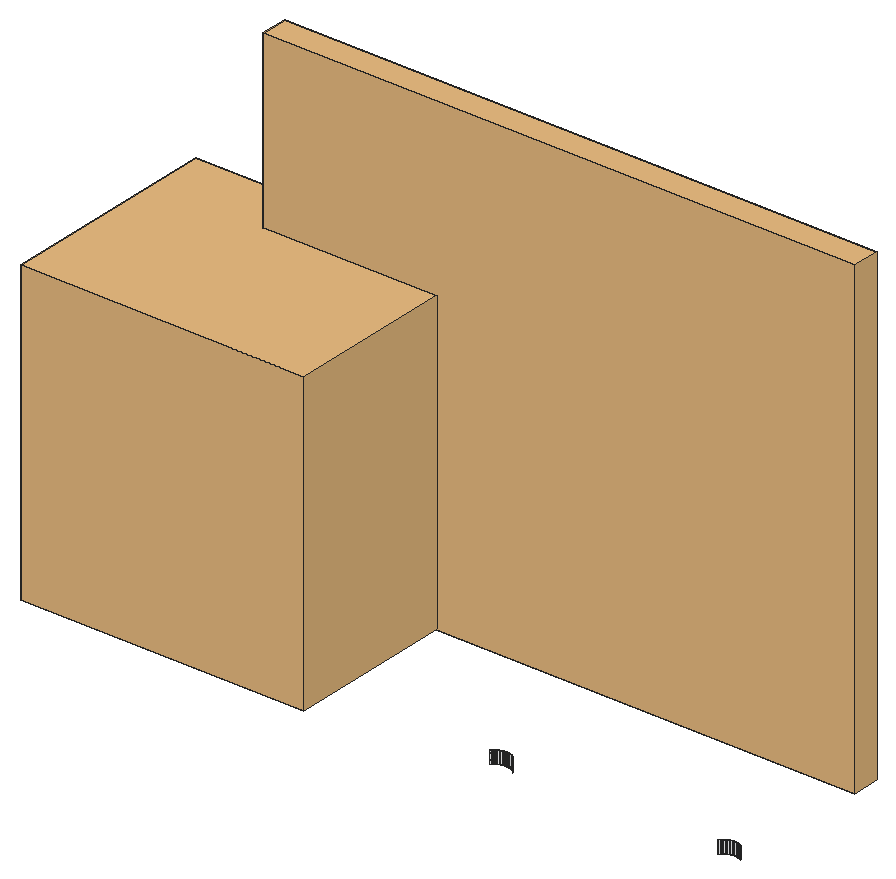
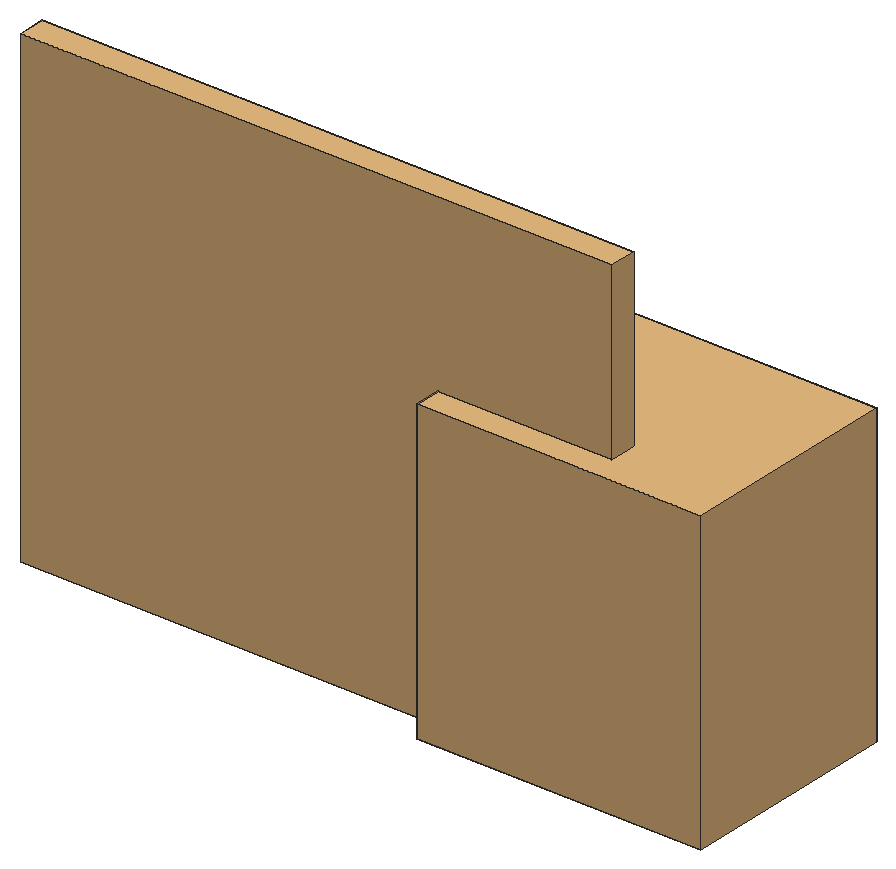
# SketchUp Ruby script. Lengths in inches.
U = 1.inch
M = Sketchup.active_model
def pt(a) = Geom::Point3d.new(a.map { |v| v * U })
def face(e, loops, mat)
  f = e.add_face(loops[0].map { |a| pt(a) })
  loops[1..].each { |l| e.add_face(l.map { |a| pt(a) }).erase! }
  f.material = f.back_material = mat if mat
  f
end
# faces: each face lists its corners as indices into pts; further lists are holes
def faces(e, pts, list, mat = nil) = list.each { |f| face(e, (f[0].is_a?(Array) ? f : [f]).map { |l| l.map { |i| pts[i] } }, mat) }
# xy, xz, yz: faces in a plane at the given z, y or x. An outline is a flat list of corners, or four numbers for a rectangle; further outlines are holes
def ring(l) = l.size == 4 ? [[l[0], l[1]], [l[2], l[1]], [l[2], l[3]], [l[0], l[3]]] : l.each_slice(2).to_a
def flat(e, list, mat, &to3) = list.each { |f| face(e, (f[0].is_a?(Array) ? f : [f]).map { |l| ring(l).map { |u, v| to3.(u, v) } }, mat) }
def xy(e, z, list, mat = nil) = flat(e, list, mat) { |x, y| [x, y, z] }
def xz(e, y, list, mat = nil) = flat(e, list, mat) { |x, z| [x, y, z] }
def yz(e, x, list, mat = nil) = flat(e, list, mat) { |y, z| [x, y, z] }
def lines(e, pts, list) = list.each { |a, b| e.add_line(pt(pts[a]), pt(pts[b])) }
# prism: a flat outline (further loops are holes) pulled along v
def prism(e, loops, v, mat = nil)
  f = face(e, loops, mat); d = Geom::Vector3d.new(v.map { |x| x * U })
  f.pushpull(f.normal.samedirection?(d) ? d.length : -d.length)
end
def box(e, o, s, mat = nil) = prism(e, [[o, [o[0] + s[0], o[1], o[2]], [o[0] + s[0], o[1] + s[1], o[2]], [o[0], o[1] + s[1], o[2]]]], [0, 0, s[2]], mat)
def at(x, y, z, deg = 0) = Geom::Transformation.translation(pt([x, y, z])) * Geom::Transformation.rotation(ORIGIN, Z_AXIS, deg.degrees)
def axes(o, x, y, z) = Geom::Transformation.new([*x, 0, *y, 0, *z, 0, *pt(o).to_a, 1])
def part(name) = M.definitions.add(name)
# library, detail: a bought-in or finely detailed component or shape, given as its bounding box
def library(name, o, s) = part(name).tap { |d| box(d.entities, o, s) }
def detail(e, o, s) = box(e.add_group.entities, o, s)
def put(e, d, t, mat = nil) = e.add_instance(d, t).tap { |i| i.material = mat if mat }
def group(e, t, mat = nil) = e.add_group.tap { |g| g.transformation = t; g.material = mat if mat }.entities
root = M.entities
M.materials.add("[Metal Seamed]").color = [36, 36, 35]
M.materials.add("[Quartz Light Grey]").color = [251, 251, 252]
c1 = library("aaa",[130.5625,121.2,0],[57.57,44.48,60.75])
c2 = library("Group\#8",[0,-4.15,0],[120,5.53,96])
xz(root,256,[[68.84,117,68.92,119.5],[68.92,117,69,119.5],[69,117,69.08,119.5],[69.08,117,69.16,119.5],[115.18,117,115.25,119.5],
  [115.25,117,115.33,119.5],[115.33,117,115.41,119.5],[115.41,117,115.49,119.5],[161.51,117,161.59,119.5],[161.59,117,161.67,119.5],
  [161.67,117,161.75,119.5],[161.75,117,161.82,119.5]],"[Quartz Light Grey]")
p = [[66.62,254.83,117],[66.67,254.89,117],[66.67,254.89,119.5],[66.62,254.83,119.5],[71.33,254.89,117],[71.38,254.83,117],
  [71.38,254.83,119.5],[71.33,254.89,119.5],[112.95,254.83,117],[113,254.89,117],[113,254.89,119.5],[112.95,254.83,119.5],
  [117.66,254.89,117],[117.71,254.83,117],[117.71,254.83,119.5],[117.66,254.89,119.5],[159.29,254.83,117],[159.34,254.89,117],
  [159.34,254.89,119.5],[159.29,254.83,119.5],[66.72,254.95,117],[66.72,254.95,119.5],[66.77,255.01,117],[66.77,255.01,119.5],
  [71.23,255.01,117],[71.28,254.95,117],[71.28,254.95,119.5],[71.23,255.01,119.5],[113.05,254.95,117],[113.05,254.95,119.5],
  [113.1,255.01,117],[113.1,255.01,119.5],[117.5625,255.01,117],[117.61,254.95,117],[117.61,254.95,119.5],[117.5625,255.01,119.5],
  [159.39,254.95,117],[159.39,254.95,119.5],[159.4375,255.01,117],[159.4375,255.01,119.5],[66.82,255.07,117],[66.82,255.07,119.5],
  [71.18,255.07,117],[71.18,255.07,119.5],[113.16,255.07,117],[113.16,255.07,119.5],[117.51,255.07,117],[117.51,255.07,119.5],
  [159.49,255.07,117],[159.49,255.07,119.5],[66.88,255.12,117],[66.88,255.12,119.5],[66.93,255.18,117],[66.93,255.18,119.5],
  [71.07,255.18,117],[71.12,255.12,117],[71.12,255.12,119.5],[71.07,255.18,119.5],[113.21,255.12,117],[113.21,255.12,119.5],
  [113.27,255.18,117],[113.27,255.18,119.5],[117.4,255.18,117],[117.45,255.12,117],[117.45,255.12,119.5],[117.4,255.18,119.5],
  [159.55,255.12,117],[159.55,255.12,119.5],[159.6,255.18,117],[159.6,255.18,119.5],[66.99,255.23,117],[66.99,255.23,119.5],
  [67.05,255.28,117],[67.05,255.28,119.5],[70.95,255.28,117],[71.01,255.23,117],[71.01,255.23,119.5],[70.95,255.28,119.5],
  [113.33,255.23,117],[113.33,255.23,119.5],[113.38,255.28,117],[113.38,255.28,119.5],[117.28,255.28,117],[117.34,255.23,117],
  [117.34,255.23,119.5],[117.28,255.28,119.5],[159.66,255.23,117],[159.66,255.23,119.5],[159.72,255.28,117],[159.72,255.28,119.5],
  [67.11,255.33,117],[67.11,255.33,119.5],[67.17,255.38,117],[67.17,255.38,119.5],[70.83,255.38,117],[70.89,255.33,117],
  [70.89,255.33,119.5],[70.83,255.38,119.5],[113.45,255.33,117],[113.45,255.33,119.5],[113.51,255.38,117],[113.51,255.38,119.5],
  [117.16,255.38,117],[117.22,255.33,117],[117.22,255.33,119.5],[117.16,255.38,119.5],[159.78,255.33,117],[159.78,255.33,119.5],
  [159.84,255.38,117],[159.84,255.38,119.5],[67.24,255.43,117],[67.24,255.43,119.5],[67.3,255.47,117],[67.3,255.47,119.5],
  [70.7,255.47,117],[70.76,255.43,117],[70.76,255.43,119.5],[70.7,255.47,119.5],[113.57,255.43,117],[113.57,255.43,119.5],
  [113.63,255.47,117],[113.63,255.47,119.5],[117.03,255.47,117],[117.1,255.43,117],[117.1,255.43,119.5],[117.03,255.47,119.5],
  [159.9,255.43,117],[159.9,255.43,119.5],[159.97,255.47,117],[159.97,255.47,119.5],[67.37,255.52,117],[67.37,255.52,119.5],
  [67.43,255.56,117],[67.43,255.56,119.5],[70.57,255.56,117],[70.63,255.52,117],[70.63,255.52,119.5],[70.57,255.56,119.5],
  [113.7,255.52,117],[113.7,255.52,119.5],[113.77,255.56,117],[113.77,255.56,119.5],[116.9,255.56,117],[116.97,255.52,117],
  [116.97,255.52,119.5],[116.9,255.56,119.5],[160.03,255.52,117],[160.03,255.52,119.5],[160.1,255.56,117],[160.1,255.56,119.5],
  [163.23,255.56,117],[163.3,255.52,117],[163.3,255.52,119.5],[163.23,255.56,119.5],[67.5,255.6,117],[67.5,255.6,119.5],
  [67.57,255.64,117],[67.57,255.64,119.5],[67.64,255.67,117],[67.64,255.67,119.5],[70.36,255.67,117],[70.43,255.64,117],
  [70.43,255.64,119.5],[70.36,255.67,119.5],[70.5,255.6,117],[70.5,255.6,119.5],[113.83,255.6,117],[113.83,255.6,119.5],
  [113.9,255.64,117],[113.9,255.64,119.5],[113.97,255.67,117],[113.97,255.67,119.5],[116.7,255.67,117],[116.76,255.64,117],
  [116.76,255.64,119.5],[116.7,255.67,119.5],[116.83,255.6,117],[116.83,255.6,119.5],[160.17,255.6,117],[160.17,255.6,119.5],
  [160.24,255.64,117],[160.24,255.64,119.5],[160.3,255.67,117],[160.3,255.67,119.5],[163.03,255.67,117],[163.1,255.64,117],
  [163.1,255.64,119.5],[163.03,255.67,119.5],[163.17,255.6,117],[163.17,255.6,119.5],[67.71,255.71,117],[67.71,255.71,119.5],
  [67.78,255.74,117],[67.78,255.74,119.5],[67.85,255.77,117],[67.85,255.77,119.5],[70.15,255.77,117],[70.22,255.74,117],
  [70.22,255.74,119.5],[70.15,255.77,119.5],[70.29,255.71,117],[70.29,255.71,119.5],[114.04,255.71,117],[114.04,255.71,119.5],
  [114.11,255.74,117],[114.11,255.74,119.5],[114.19,255.77,117],[114.19,255.77,119.5],[116.48,255.77,117],[116.55,255.74,117],
  [116.55,255.74,119.5],[116.48,255.77,119.5],[116.625,255.71,117],[116.625,255.71,119.5],[160.375,255.71,117],[160.375,255.71,119.5],
  [160.45,255.74,117],[160.45,255.74,119.5],[160.52,255.77,117],[160.52,255.77,119.5],[162.81,255.77,117],[162.89,255.74,117],
  [162.89,255.74,119.5],[162.81,255.77,119.5],[162.96,255.71,117],[162.96,255.71,119.5],[67.92,255.8,117],[67.92,255.8,119.5],
  [68,255.83,117],[68,255.83,119.5],[68.07,255.85,117],[68.07,255.85,119.5],[69.93,255.85,117],[70,255.83,117],
  [70,255.83,119.5],[69.93,255.85,119.5],[70.08,255.8,117],[70.08,255.8,119.5],[114.26,255.8,117],[114.26,255.8,119.5],
  [114.33,255.83,117],[114.33,255.83,119.5],[114.41,255.85,117],[114.41,255.85,119.5],[116.26,255.85,117],[116.33,255.83,117],
  [116.33,255.83,119.5],[116.26,255.85,119.5],[116.41,255.8,117],[116.41,255.8,119.5],[160.59,255.8,117],[160.59,255.8,119.5],
  [160.67,255.83,117],[160.67,255.83,119.5],[160.74,255.85,117],[160.74,255.85,119.5],[162.59,255.85,117],[162.67,255.83,117],
  [162.67,255.83,119.5],[162.59,255.85,119.5],[162.74,255.8,117],[162.74,255.8,119.5],[68.15,255.875,117],[68.15,255.875,119.5],
  [68.22,255.9,117],[68.22,255.9,119.5],[68.3,255.92,117],[68.3,255.92,119.5],[68.375,255.93,117],[68.375,255.93,119.5],
  [68.45,255.95,117],[68.45,255.95,119.5],[68.53,255.96,117],[68.53,255.96,119.5],[69.47,255.96,117],[69.55,255.95,117],
  [69.55,255.95,119.5],[69.47,255.96,119.5],[69.625,255.93,117],[69.625,255.93,119.5],[69.7,255.92,117],[69.7,255.92,119.5],
  [69.78,255.9,117],[69.78,255.9,119.5],[69.85,255.875,117],[69.85,255.875,119.5],[114.48,255.875,117],[114.48,255.875,119.5],
  [114.56,255.9,117],[114.56,255.9,119.5],[114.63,255.92,117],[114.63,255.92,119.5],[114.71,255.93,117],[114.71,255.93,119.5],
  [114.79,255.95,117],[114.79,255.95,119.5],[114.86,255.96,117],[114.86,255.96,119.5],[115.8,255.96,117],[115.88,255.95,117],
  [115.88,255.95,119.5],[115.8,255.96,119.5],[115.96,255.93,117],[115.96,255.93,119.5],[116.03,255.92,117],[116.03,255.92,119.5],
  [116.11,255.9,117],[116.11,255.9,119.5],[116.19,255.875,117],[116.19,255.875,119.5],[160.81,255.875,117],[160.81,255.875,119.5],
  [160.89,255.9,117],[160.89,255.9,119.5],[160.97,255.92,117],[160.97,255.92,119.5],[161.04,255.93,117],[161.04,255.93,119.5],
  [161.12,255.95,117],[161.12,255.95,119.5],[161.2,255.96,117],[161.2,255.96,119.5],[162.14,255.96,117],[162.21,255.95,117],
  [162.21,255.95,119.5],[162.14,255.96,119.5],[162.29,255.93,117],[162.29,255.93,119.5],[162.37,255.92,117],[162.37,255.92,119.5],
  [162.44,255.9,117],[162.44,255.9,119.5],[162.52,255.875,117],[162.52,255.875,119.5],[68.61,255.97,117],[68.61,255.97,119.5],
  [68.6875,255.98,117],[68.6875,255.98,119.5],[68.76,255.99,117],[68.76,255.99,119.5],[68.84,256,117],[68.84,256,119.5],
  [69.16,256,117],[69.24,255.99,117],[69.24,255.99,119.5],[69.16,256,119.5],[69.3125,255.98,117],[69.3125,255.98,119.5],
  [69.39,255.97,117],[69.39,255.97,119.5],[114.94,255.97,117],[114.94,255.97,119.5],[115.02,255.98,117],[115.02,255.98,119.5],
  [115.1,255.99,117],[115.1,255.99,119.5],[115.18,256,117],[115.18,256,119.5],[115.49,256,117],[115.57,255.99,117],
  [115.57,255.99,119.5],[115.49,256,119.5],[115.65,255.98,117],[115.65,255.98,119.5],[115.72,255.97,117],[115.72,255.97,119.5],
  [161.28,255.97,117],[161.28,255.97,119.5],[161.35,255.98,117],[161.35,255.98,119.5],[161.43,255.99,117],[161.43,255.99,119.5],
  [161.51,256,117],[161.51,256,119.5],[161.82,256,117],[161.9,255.99,117],[161.9,255.99,119.5],[161.82,256,119.5],
  [161.98,255.98,117],[161.98,255.98,119.5],[162.06,255.97,117],[162.06,255.97,119.5],[54,271,126],[174,271,126]]
faces(root,p,[[0,1,2,3],[4,5,6,7],[8,9,10,11],[12,13,14,15],[16,17,18,19],[1,20,21,2],[20,22,23,21],[24,25,26,27],
  [25,4,7,26],[9,28,29,10],[28,30,31,29],[32,33,34,35],[33,12,15,34],[17,36,37,18],[36,38,39,37],[22,40,41,23],
  [42,24,27,43],[30,44,45,31],[46,32,35,47],[38,48,49,39],[40,50,51,41],[50,52,53,51],[54,55,56,57],[55,42,43,56],
  [44,58,59,45],[58,60,61,59],[62,63,64,65],[63,46,47,64],[48,66,67,49],[66,68,69,67],[52,70,71,53],[70,72,73,71],
  [74,75,76,77],[75,54,57,76],[60,78,79,61],[78,80,81,79],[82,83,84,85],[83,62,65,84],[68,86,87,69],[86,88,89,87],
  [72,90,91,73],[90,92,93,91],[94,95,96,97],[95,74,77,96],[80,98,99,81],[98,100,101,99],[102,103,104,105],[103,82,85,104],
  [88,106,107,89],[106,108,109,107],[92,110,111,93],[110,112,113,111],[114,115,116,117],[115,94,97,116],[100,118,119,101],[118,120,121,119],
  [122,123,124,125],[123,102,105,124],[108,126,127,109],[126,128,129,127],[112,130,131,113],[130,132,133,131],[134,135,136,137],[135,114,117,136],
  [120,138,139,121],[138,140,141,139],[142,143,144,145],[143,122,125,144],[128,146,147,129],[146,148,149,147],[150,151,152,153],[132,154,155,133],
  [154,156,157,155],[156,158,159,157],[160,161,162,163],[161,164,165,162],[164,134,137,165],[140,166,167,141],[166,168,169,167],[168,170,171,169],
  [172,173,174,175],[173,176,177,174],[176,142,145,177],[148,178,179,149],[178,180,181,179],[180,182,183,181],[184,185,186,187],[185,188,189,186],
  [188,150,153,189],[158,190,191,159],[190,192,193,191],[192,194,195,193],[196,197,198,199],[197,200,201,198],[200,160,163,201],[170,202,203,171],
  [202,204,205,203],[204,206,207,205],[208,209,210,211],[209,212,213,210],[212,172,175,213],[182,214,215,183],[214,216,217,215],[216,218,219,217],
  [220,221,222,223],[221,224,225,222],[224,184,187,225],[194,226,227,195],[226,228,229,227],[228,230,231,229],[232,233,234,235],[233,236,237,234],
  [236,196,199,237],[206,238,239,207],[238,240,241,239],[240,242,243,241],[244,245,246,247],[245,248,249,246],[248,208,211,249],[218,250,251,219],
  [250,252,253,251],[252,254,255,253],[256,257,258,259],[257,260,261,258],[260,220,223,261],[230,262,263,231],[262,264,265,263],[264,266,267,265],
  [266,268,269,267],[268,270,271,269],[270,272,273,271],[274,275,276,277],[275,278,279,276],[278,280,281,279],[280,282,283,281],[282,284,285,283],
  [284,232,235,285],[242,286,287,243],[286,288,289,287],[288,290,291,289],[290,292,293,291],[292,294,295,293],[294,296,297,295],[298,299,300,301],
  [299,302,303,300],[302,304,305,303],[304,306,307,305],[306,308,309,307],[308,244,247,309],[254,310,311,255],[310,312,313,311],[312,314,315,313],
  [314,316,317,315],[316,318,319,317],[318,320,321,319],[322,323,324,325],[323,326,327,324],[326,328,329,327],[328,330,331,329],[330,332,333,331],
  [332,256,259,333],[272,334,335,273],[334,336,337,335],[336,338,339,337],[338,340,341,339],[342,343,344,345],[343,346,347,344],[346,348,349,347],
  [348,274,277,349],[296,350,351,297],[350,352,353,351],[352,354,355,353],[354,356,357,355],[358,359,360,361],[359,362,363,360],[362,364,365,363],
  [364,298,301,365],[320,366,367,321],[366,368,369,367],[368,370,371,369],[370,372,373,371],[374,375,376,377],[375,378,379,376],[378,380,381,379],
  [380,322,325,381]],"[Quartz Light Grey]")
lines(root,p,[[382,383]])
put(root,c1,at(-98.92,116.21,126))
put(root,c2,at(54,275.15,126),"[Metal Seamed]")
